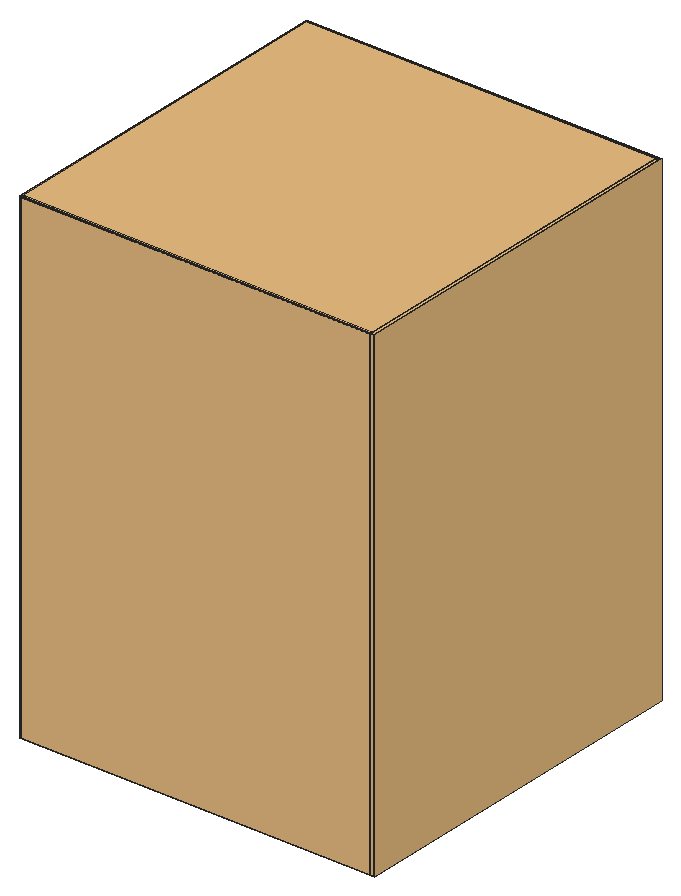
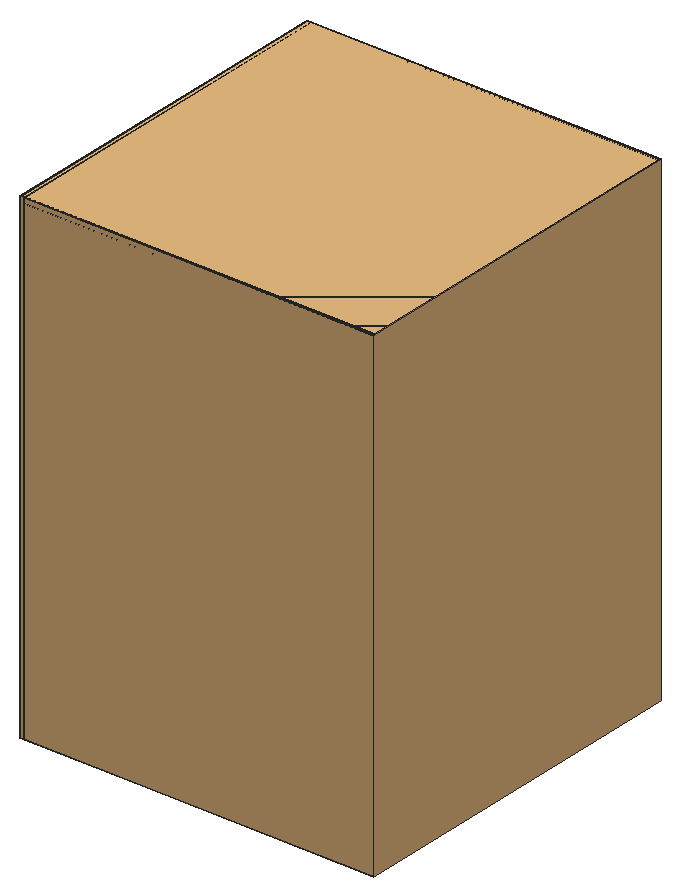
# SketchUp Ruby script. Lengths in inches.
U = 1.inch
M = Sketchup.active_model
def pt(a) = Geom::Point3d.new(a.map { |v| v * U })
def face(e, loops, mat)
  f = e.add_face(loops[0].map { |a| pt(a) })
  loops[1..].each { |l| e.add_face(l.map { |a| pt(a) }).erase! }
  f.material = f.back_material = mat if mat
  f
end
# faces: each face lists its corners as indices into pts; further lists are holes
def faces(e, pts, list, mat = nil) = list.each { |f| face(e, (f[0].is_a?(Array) ? f : [f]).map { |l| l.map { |i| pts[i] } }, mat) }
# xy, xz, yz: faces in a plane at the given z, y or x. An outline is a flat list of corners, or four numbers for a rectangle; further outlines are holes
def ring(l) = l.size == 4 ? [[l[0], l[1]], [l[2], l[1]], [l[2], l[3]], [l[0], l[3]]] : l.each_slice(2).to_a
def flat(e, list, mat, &to3) = list.each { |f| face(e, (f[0].is_a?(Array) ? f : [f]).map { |l| ring(l).map { |u, v| to3.(u, v) } }, mat) }
def xy(e, z, list, mat = nil) = flat(e, list, mat) { |x, y| [x, y, z] }
def xz(e, y, list, mat = nil) = flat(e, list, mat) { |x, z| [x, y, z] }
def yz(e, x, list, mat = nil) = flat(e, list, mat) { |y, z| [x, y, z] }
def lines(e, pts, list) = list.each { |a, b| e.add_line(pt(pts[a]), pt(pts[b])) }
# prism: a flat outline (further loops are holes) pulled along v
def prism(e, loops, v, mat = nil)
  f = face(e, loops, mat); d = Geom::Vector3d.new(v.map { |x| x * U })
  f.pushpull(f.normal.samedirection?(d) ? d.length : -d.length)
end
def box(e, o, s, mat = nil) = prism(e, [[o, [o[0] + s[0], o[1], o[2]], [o[0] + s[0], o[1] + s[1], o[2]], [o[0], o[1] + s[1], o[2]]]], [0, 0, s[2]], mat)
def at(x, y, z, deg = 0) = Geom::Transformation.translation(pt([x, y, z])) * Geom::Transformation.rotation(ORIGIN, Z_AXIS, deg.degrees)
def axes(o, x, y, z) = Geom::Transformation.new([*x, 0, *y, 0, *z, 0, *pt(o).to_a, 1])
def part(name) = M.definitions.add(name)
# library, detail: a bought-in or finely detailed component or shape, given as its bounding box
def library(name, o, s) = part(name).tap { |d| box(d.entities, o, s) }
def detail(e, o, s) = box(e.add_group.entities, o, s)
def put(e, d, t, mat = nil) = e.add_instance(d, t).tap { |i| i.material = mat if mat }
def group(e, t, mat = nil) = e.add_group.tap { |g| g.transformation = t; g.material = mat if mat }.entities
root = M.entities
M.materials.add("green").color = [174, 139, 102]
M.materials.add("vio").color = [206, 114, 100]
c1 = library("3DGeom~69_Defintion",[-21.55,-528.54,-60.47],[37.16,1000,121.53])
c2 = library("3DGeom~72_Defintion",[-21.55,-528.54,-60.94],[37.16,1000,122])
c3 = part("3DGeom~65_Defintion")
p = [[7.52,100.36,-59.99],[8.92,100.38,-59.73],[8.93,76.8125,-54.81],[7.56,76.76,-55.0625],[3.04,143.42,-39.85],[7.31,123.06,-53.64],
  [5.89,123.05,-53.91],[4.49,143.43,-39.59],[14.26,515.51,-51.87],[10.45,459.87,-31.05],[8.63,459.92,-31.36],[16.125,515.46,-51.55],
  [6.62,54.24,-42.53],[6.5,32.65,-26.04],[5.18,32.59,-26.27],[7.96,54.3,-42.28],[9.77,-132.64,-34.95],[8.22,-159.71,-27.66],
  [7.13,-159.66,-27.85],[10.89,-132.67,-34.76],[9.125,-89.93,-24.57],[11.4,-109.33,-33.07],[10.25,-109.31,-33.26],[10.29,-89.9375,-24.36],
  [-3.2,185.09,-5.2],[1.25,163.47,-22.06],[-0.23,163.47,-22.32],[-1.7,185.08,-4.93],[3.93,408.18,-14.71],[1.85,360.26,-1.6],
  [0.14,360.3,-1.9],[5.6875,408.13,-14.4],[2.8125,-189.42,-14.64],[-1.36,-221.25,2.05],[-2.375,-221.2,1.87],[3.87,-189.48,-14.46],
  [4.88,-58.05,-0.94],[8.29,-73.3125,-12.4],[7.1,-73.3125,-12.62],[6.08,-58.04,-0.72],[3.69,11.76,-9.89],[3.86,-8.04,3.3],
  [2.59,-8.09,3.07],[4.99,11.82,-9.66],[-2.72,316.3,7.07],[-3.06,276.15,12.48],[-4.67,276.18,12.21],[-1.0625,316.27,7.35],
  [2.27,-26.52,9.24],[4.32,-42.88,7.46],[3.09,-42.9,7.22],[3.52,-26.49,9.47],[-5.7,239.97,13.5],[-3.7,209.94,8.14],
  [-5.24,209.96,7.88],[-4.13,239.94,13.77],[-7.64,-254.13,18.93],[-11.22,-287.3125,33.93],[-12.17,-287.28,33.77],[-6.65,-254.18,19.09],
  [-15.18,-319.65,43.67],[-15.95,-351.88,49.35],[-16.84,-351.87,49.21],[-14.26,-319.67,43.82],[-17.57,-450.77,52.97],[-15.66,-484.48,50.06],
  [-16.4,-484.49,49.94],[-16.79,-450.76,53.09],[-17.79,-384.46,52.6],[-17.22,-417.43,53.99],[-18.03,-417.43,53.86],[-16.94,-384.47,52.74]]
faces(c3.entities,p,[[0,1,2],[0,2,3],[4,5,6],[4,7,5],[8,9,10],[8,11,9],[12,13,14],[12,15,13],
  [16,17,18],[16,19,17],[20,21,22],[20,23,21],[24,25,26],[24,27,25],[28,29,30],[28,31,29],
  [32,33,34],[32,35,33],[36,37,38],[36,39,37],[40,41,42],[40,43,41],[44,45,46],[44,47,45],
  [48,49,50],[48,51,49],[52,53,54],[52,55,53],[56,57,58],[56,59,57],[60,61,62],[60,63,61],
  [64,65,66],[64,67,65],[68,69,70],[68,71,69]],"green")
c4 = part("3DGeom~68_Defintion")
p = [[6.16,100.31,-59.87],[7.52,100.34,-59.98],[7.56,76.74,-55.05],[6.21,76.79,-54.96],[8.91,100.36,-59.72],[10.17,76.95,-54.21],
  [8.92,76.8,-54.8],[10.1875,100.38,-59.09],[1.63,143.2,-39.79],[5.89,123.02,-53.9],[4.5,122.88,-53.81],[3.04,143.39,-39.84],
  [4.48,143.4,-39.58],[8.62,122.92,-53.03],[7.31,123.04,-53.63],[5.83,143.21,-39.01],[12.45,515.58,-51.71],[14.26,515.4,-51.86],
  [8.63,459.82,-31.36],[6.87,459.98,-31.21],[16.12,515.35,-51.54],[12.12,459.84,-30.29],[10.44,459.77,-31.05],[17.84,515.4375,-50.76],
  [5.3,54.32,-42.45],[6.61,54.23,-42.52],[5.18,32.58,-26.27],[3.89,32.68,-26.21],[7.96,54.29,-42.28],[7.71,32.88,-25.52],
  [6.5,32.65,-26.03],[9.1875,54.5,-41.73],[7.71,32.88,-25.52],[8.67,-132.56,-34.83],[9.76,-132.61,-34.94],[7.13,-159.63,-27.84],
  [10.89,-132.65,-34.76],[9.23,-159.65,-27.2],[8.22,-159.68,-27.66],[6.07,-159.51,-27.75],[11.93,-132.65,-34.28],[7.99,-90.02,-24.49],
  [9.125,-89.91,-24.56],[10.25,-109.28,-33.26],[9.13,-109.32,-33.15],[10.29,-89.92,-24.36],[12.45,-109.39,-32.58],[11.4,-109.31,-33.07],
  [11.37,-90.05,-23.89],[-4.67,184.89,-5.11],[-0.23,163.4375,-22.32],[-1.66,163.24,-22.26],[-3.2,185.05,-5.19],[-1.7,185.04,-4.93],
  [2.62,163.24,-21.49],[1.25,163.44,-22.05],[-0.3,184.86,-4.34],[2.62,163.24,-21.49],[2.21,408.23,-14.55],[3.93,408.09,-14.7],
  [0.14,360.23,-1.9],[1.79,-189.24,-14.5625],[-2.375,-221.15,1.87],[-3.36,-221.01,1.9375],[2.8125,-189.38,-14.64],[-1.53,360.34,-1.74],
  [3.87,-189.4375,-14.46],[-0.41,-221.16,2.46],[-1.36,-221.21,2.05],[4.84,-189.4,-14.02],[5.6875,408.05,-14.4],[3.43,360.23,-0.88],
  [1.85,360.1875,-1.6],[7.3125,408.11,-13.66],[3.71,-58.1875,-0.89],[7.1,-73.3,-12.61],[5.95,-73.45,-12.5625],[4.88,-58.04,-0.94],
  [6.08,-58.03,-0.72],[9.39,-73.45,-11.9375],[8.29,-73.3,-12.4],[7.2,-58.16,-0.23],[9.39,-73.45,-11.9375],[2.43,11.85,-9.83],
  [3.69,11.75,-9.89],[2.59,-8.09,3.07],[1.34,-8.02,3.15],[4.99,11.82,-9.66],[5.02,-7.87,3.83],[3.86,-8.04,3.3],
  [6.17,12.03,-9.14],[5.02,-7.87,3.83],[-4.34,316.32,7.22],[-2.72,316.23,7.07],[-4.67,276.12,12.2],[1.05,-26.51,9.34],
  [3.09,-42.89,7.22],[1.89,-42.99,7.31],[2.27,-26.51,9.24],[-6.24,276.17,12.36],[-1.0625,316.2,7.35],[-1.57,276.09,13.17],
  [-3.06,276.09,12.48],[0.47,316.22,8.0625],[3.52,-26.49,9.47],[5.44,-42.94,7.99],[4.32,-42.875,7.45],[-7.22,239.93,13.65],
  [-5.23,209.91,7.88],[-6.73,209.82,8.01],[-5.69,239.92,13.5],[4.65,-26.43,10.03],[-4.13,239.89,13.76],[-2.29,209.78,8.79],
  [-3.7,209.9,8.14],[-2.7,239.86,14.43],[-8.59,-253.95,18.99],[-7.64,-254.08,18.92],[-12.17,-287.22,33.76],[-13.09,-287.11,33.84],
  [-6.65,-254.125,19.09],[-10.33,-287.22,34.3125],[-11.21,-287.25,33.92],[-5.74,-254.08,19.49],[-16.07,-319.53,43.75],[-15.17,-319.59,43.66],
  [-16.83,-351.79,49.2],[-17.69,-351.76,49.29],[-14.26,-319.61,43.81],[-15.14,-351.79,49.71],[-15.95,-351.81,49.34],[-13.41,-319.59,44.19],
  [-18.32,-450.69,53.04],[-17.57,-450.68,52.96],[-16.4,-484.39,49.93],[-17.12,-484.42,50.01],[-16.79,-450.67,53.08],[-14.97,-484.38,50.36],
  [-15.66,-484.375,50.05],[-16.08,-450.67,53.41],[-18.61,-384.37,52.68],[-17.78,-384.38,52.59],[-18.03,-417.34,53.85],[-18.82,-417.34,53.93],
  [-16.9375,-384.39,52.73],[-16.47,-417.34,54.32],[-17.22,-417.34,53.98],[-16.16,-384.38,53.08]]
faces(c4.entities,p,[[0,1,2],[0,2,3],[4,5,6],[4,7,5],[8,9,10],[8,11,9],[12,13,14],[12,15,13],
  [16,17,18],[16,18,19],[20,21,22],[20,23,21],[24,25,26],[24,26,27],[28,29,30],[28,31,32],
  [33,34,35],[36,37,38],[33,35,39],[36,40,37],[41,42,43],[41,43,44],[45,46,47],[45,48,46],
  [49,50,51],[49,52,50],[53,54,55],[53,56,57],[58,59,60],[61,62,63],[61,64,62],[58,60,65],
  [66,67,68],[66,69,67],[70,71,72],[70,73,71],[74,75,76],[74,77,75],[78,79,80],[78,81,82],
  [83,84,85],[83,85,86],[87,88,89],[87,90,91],[92,93,94],[95,96,97],[95,98,96],[92,94,99],
  [100,101,102],[100,103,101],[104,105,106],[107,108,109],[107,110,108],[104,111,105],[112,113,114],[112,115,113],
  [116,117,118],[116,118,119],[120,121,122],[120,123,121],[124,125,126],[124,126,127],[128,129,130],[128,131,129],
  [132,133,134],[132,134,135],[136,137,138],[136,139,137],[140,141,142],[140,142,143],[144,145,146],[144,147,145]],"green")
c5 = library("3DGeom~67_Defintion",[-21.08,-482.92,-59.16],[42.16,1000,118.9])
c6 = library("3DGeom~71_Defintion",[-21.08,-482.92,-59.62],[42.16,1000,119.36])
c7 = part("3DGeom~73_Defintion")
p = [[11.99,496.51,-49.8],[15.53,496.29,-49.63],[13.73,496.34,-49.94],[11.99,496.51,-49.8],[19.55,496.875,-46.43],[15.53,496.29,-49.63],
  [8.98,497.16,-48.31],[19.55,496.875,-46.43],[11.99,496.51,-49.8],[8.98,497.16,-48.31],[11.99,496.51,-49.8],[10.38,496.79,-49.24],
  [15.53,496.29,-49.63],[19.55,496.875,-46.43],[18.54,496.57,-47.79],[15.53,496.29,-49.63],[18.54,496.57,-47.79],[17.18,496.37,-48.89],
  [7.13,498.09,-45.48],[19.55,496.875,-46.43],[8.98,497.16,-48.31],[7.13,498.09,-45.48],[8.98,497.16,-48.31],[7.87,497.6,-47.04],
  [7.06,499.03,-42.12],[19.55,496.875,-46.43],[7.13,498.09,-45.48],[8.7,499.72,-39.2],[19.55,496.875,-46.43],[7.06,499.03,-42.12],
  [11.72,500,-37.36],[19.55,496.875,-46.43],[8.7,499.72,-39.2],[15.25,499.78,-37.19],[19.55,496.875,-46.43],[11.72,500,-37.36],
  [20.18,497.26,-44.875],[19.55,496.875,-46.43],[15.25,499.78,-37.19],[7.06,499.03,-42.12],[7.13,498.09,-45.48],[6.86,498.58,-43.78],
  [20.18,497.26,-44.875],[15.25,499.78,-37.19],[16.86,499.5,-37.75],[19.37,498.7,-39.95],[20.18,497.26,-44.875],[16.86,499.5,-37.75],
  [20.11,498.2,-41.51],[20.18,497.26,-44.875],[19.37,498.7,-39.95],[20.11,498.2,-41.51],[20.38,497.71,-43.21],[20.18,497.26,-44.875],
  [8.7,499.72,-39.2],[7.06,499.03,-42.12],[7.6875,499.41,-40.5625],[19.37,498.7,-39.95],[16.86,499.5,-37.75],[18.26,499.13,-38.68],
  [11.72,500,-37.36],[8.7,499.72,-39.2],[10.0625,499.92,-38.11],[15.25,499.78,-37.19],[11.72,500,-37.36],[13.51,499.95,-37.05],
  [-14.64,-499.34,43.17],[-13.98,-499.3,43.1],[-13.3,-499.28,43.21],[-15.79,-499.47,43.77],[-15.26,-499.4,43.4],[-14.64,-499.34,43.17],
  [-15.79,-499.47,43.77],[-14.64,-499.34,43.17],[-11.78,-499.375,44.44],[-14.64,-499.34,43.17],[-13.3,-499.28,43.21],[-11.78,-499.375,44.44],
  [-13.3,-499.28,43.21],[-12.16,-499.32,43.91],[-11.78,-499.375,44.44],[-13.3,-499.28,43.21],[-12.68,-499.29,43.49],[-12.16,-499.32,43.91],
  [-16.49,-499.66,44.89],[-16.21,-499.56,44.28],[-15.79,-499.47,43.77],[-16.49,-499.66,44.89],[-15.79,-499.47,43.77],[-11.78,-499.375,44.44],
  [-15.9,-499.96,47.36],[-16.52,-499.84,46.22],[-11.78,-499.375,44.44],[-14.76,-500,48.06],[-15.9,-499.96,47.36],[-11.78,-499.375,44.44],
  [-13.42,-499.94,48.1],[-14.76,-500,48.06],[-11.78,-499.375,44.44],[-11.54,-499.44,45.05],[-13.42,-499.94,48.1],[-11.78,-499.375,44.44],
  [-16.52,-499.84,46.22],[-16.49,-499.66,44.89],[-11.78,-499.375,44.44],[-16.52,-499.84,46.22],[-16.6,-499.75,45.57],[-16.49,-499.66,44.89],
  [-11.54,-499.44,45.05],[-12.81,-499.88,47.87],[-13.42,-499.94,48.1],[-11.85,-499.72,46.99],[-12.81,-499.88,47.87],[-11.54,-499.44,45.05],
  [-11.54,-499.44,45.05],[-11.57,-499.625,46.375],[-11.85,-499.72,46.99],[-11.54,-499.44,45.05],[-11.47,-499.53,45.7],[-11.57,-499.625,46.375],
  [-15.9,-499.96,47.36],[-16.28,-499.91,46.83],[-16.52,-499.84,46.22],[-11.85,-499.72,46.99],[-12.28,-499.81,47.5],[-12.81,-499.88,47.87],
  [-14.76,-500,48.06],[-15.39,-499.99,47.78],[-15.9,-499.96,47.36],[-13.42,-499.94,48.1],[-14.08,-499.98,48.17],[-14.76,-500,48.06]]
faces(c7.entities,p,[[0,1,2],[3,4,5],[6,7,8],[9,10,11],[12,13,14],[15,16,17],[18,19,20],[21,22,23],
  [24,25,26],[27,28,29],[30,31,32],[33,34,35],[36,37,38],[39,40,41],[42,43,44],[45,46,47],
  [48,49,50],[51,52,53],[54,55,56],[57,58,59],[60,61,62],[63,64,65],[66,67,68],[69,70,71],
  [72,73,74],[75,76,77],[78,79,80],[81,82,83],[84,85,86],[87,88,89],[90,91,92],[93,94,95],
  [96,97,98],[99,100,101],[102,103,104],[105,106,107],[108,109,110],[111,112,113],[114,115,116],[117,118,119],
  [120,121,122],[123,124,125],[126,127,128],[129,130,131]],"green")
c8 = library("3DGeom~1_Defintion",[-369.63,-500,-363.56],[735.81,1000,728.59])
c9 = library("3DGeom~2_Defintion",[-372.64,-496.69,-369.59],[746.89,1000,738.52])
c10 = library("3DGeom~3_Defintion",[-370.01,-499.5,-356.78],[740.02,1000,722.18])
c11 = library("3DGeom~4_Defintion",[-369.63,-500,-365.03],[739.26,1000,729.3])
c12 = library("3DGeom~5_Defintion",[-370.16,-506.05,-369.45],[742.08,1000,738.24])
c13 = library("3DGeom~6_Defintion",[-367.72,-498.8,-365.91],[735.57,1000,731.94])
c14 = part("3DGeom~242_Defintion")
p = [[-230.85,-87.93,-431.85],[22.11,-101.53,-485.51],[16.43,-294.21,-360.73],[264.23,-254.8,-301.01],[16.43,-294.21,-360.73],[269.15,-87.93,-409.08],
  [264.23,-254.8,-301.01],[-231.0625,102.5,-427.26],[21.87,118.36,-480.21],[-230.85,-87.93,-431.85],[268.9375,102.5,-404.49],[-236.35,265.46,-311.23],
  [15.77,306.53,-346.23],[-236.35,265.46,-311.23],[-230.85,-87.93,-431.85],[16.43,-294.21,-360.73],[-235.78,-254.8,-323.78],[-421.96,-50.77,-262.47],
  [-230.85,-87.93,-431.85],[-235.78,-254.8,-323.78],[-422.08,59.18,-259.82],[-230.85,-87.93,-431.85],[-422.08,59.18,-259.82],[-230.85,-87.93,-431.85],
  [-421.96,-50.77,-262.47],[-425.13,153.27,-192.83],[-231.0625,102.5,-427.26],[-422.08,59.18,-259.82],[-236.35,265.46,-311.23],[-231.0625,102.5,-427.26],
  [269.15,-87.93,-409.08],[441.23,-147.11,-160.65],[264.23,-254.8,-301.01],[269.15,-87.93,-409.08],[444.07,-50.76,-223.04],[268.9375,102.5,-404.49],
  [269.15,-87.93,-409.08],[268.9375,102.5,-404.49],[443.95,59.18,-220.39],[263.65,265.47,-288.46],[268.9375,102.5,-404.49],[263.65,265.47,-288.46],
  [-235.78,-254.8,-323.78],[16.43,-294.21,-360.73],[6.34,-408.0625,-139.28],[255.49,-353.39,-109.24],[264.23,-254.8,-301.01],[-245.29,357.3,-114.86],
  [15.77,306.53,-346.23],[-236.35,265.46,-311.23],[5.44,412.57,-119.48],[263.65,265.47,-288.46],[15.77,306.53,-346.23],[-245.29,357.3,-114.86],
  [15.77,306.53,-346.23],[-235.78,-254.8,-323.78],[-244.51,-353.39,-132.01],[-424.8,-147.11,-200.08],[-244.51,-353.39,-132.01],[-430.29,206.29,-79.46],
  [-245.29,357.3,-114.86],[264.23,-254.8,-301.01],[436.18,-204.03,-49.92],[255.49,-353.39,-109.24],[264.23,-254.8,-301.01],[263.65,265.47,-288.46],
  [440.9,153.27,-153.4],[254.71,357.3,-92.09],[263.65,265.47,-288.46],[254.71,357.3,-92.09],[263.65,265.47,-288.46],[-500,0,-22.77],
  [500,0,22.77],[-429.84,-204.03,-89.36],[435.73,206.29,-40.02],[254.71,357.3,-92.09],[-244.51,-353.39,-132.01],[-5.44,-412.57,119.48],
  [245.29,-357.3,114.86],[-244.51,-353.39,-132.01],[-254.71,-357.3,92.09],[-254.71,-357.3,92.09],[-255.49,353.39,109.24],[-6.34,408.0625,139.28],
  [-255.49,353.39,109.24],[-245.29,357.3,-114.86],[-436.18,204.03,49.92],[-255.49,353.39,109.24],[255.49,-353.39,-109.24],[430.29,-206.29,79.46],
  [245.29,-357.3,114.86],[255.49,-353.39,-109.24],[244.51,353.39,132.01],[254.71,357.3,-92.09],[244.51,353.39,132.01],[-435.73,-206.29,40.02],
  [429.84,204.03,89.36],[244.51,353.39,132.01],[-440.9,-153.27,153.4],[-443.95,-59.18,220.39],[-444.07,50.77,223.04],[-441.23,147.11,160.65],
  [425.13,-153.27,192.83],[422.08,-59.18,259.82],[421.96,50.77,262.47],[424.8,147.11,200.08],[-263.65,-265.47,288.46],[245.29,-357.3,114.86],
  [235.78,254.8,323.78],[235.78,254.8,323.78],[244.51,353.39,132.01],[-254.71,-357.3,92.09],[-15.77,-306.53,346.23],[-254.71,-357.3,92.09],
  [-15.77,-306.53,346.23],[-263.65,-265.47,288.46],[-264.22,254.8,301.01],[-264.22,254.8,301.01],[-255.49,353.39,109.24],[236.35,-265.47,311.23],
  [245.29,-357.3,114.86],[236.35,-265.47,311.23],[236.35,-265.47,311.23],[-15.77,-306.53,346.23],[-16.43,294.21,360.73],[235.78,254.8,323.78],
  [-264.22,254.8,301.01],[-268.9375,-102.5,404.49],[236.35,-265.47,311.23],[230.85,87.93,431.85],[230.85,87.93,431.85],[235.78,254.8,323.78],
  [-269.15,87.93,409.08],[236.35,-265.47,311.23],[231.0625,-102.5,427.26],[231.0625,-102.5,427.26],[422.08,-59.18,259.82],[421.96,50.77,262.47],
  [421.96,50.77,262.47],[230.85,87.93,431.85],[-263.65,-265.47,288.46],[-15.77,-306.53,346.23],[-21.87,-118.36,480.21],[-263.65,-265.47,288.46],
  [-268.9375,-102.5,404.49],[-269.15,87.93,409.08],[-16.43,294.21,360.73],[-264.22,254.8,301.01],[236.35,-265.47,311.23],[-22.11,101.53,485.51],
  [235.78,254.8,323.78],[235.78,254.8,323.78],[-16.43,294.21,360.73],[-269.15,87.93,409.08],[-16.43,294.21,360.73],[-268.9375,-102.5,404.49],
  [-268.9375,-102.5,404.49],[-269.15,87.93,409.08]]
faces(c14.entities,p,[[0,1,2],[1,3,4],[1,5,6],[7,8,1],[7,1,9],[8,5,1],[8,10,5],[11,8,7],
  [12,10,8],[13,12,8],[14,15,16],[17,18,19],[20,7,21],[22,23,24],[25,26,27],[25,28,29],
  [30,31,32],[33,34,31],[35,34,36],[37,38,34],[39,38,40],[12,41,10],[42,43,44],[43,45,44],
  [43,46,45],[47,48,49],[50,51,52],[53,50,54],[55,44,56],[57,19,58],[17,19,57],[59,28,25],
  [59,60,28],[61,62,63],[64,31,62],[65,66,38],[67,66,68],[50,69,70],[17,57,71],[27,17,71],
  [25,27,71],[31,34,72],[34,38,72],[38,66,72],[57,58,73],[57,73,71],[59,25,71],[62,31,72],
  [66,74,72],[75,74,66],[76,44,77],[44,78,77],[44,45,78],[79,77,80],[73,58,81],[82,83,50],
  [84,50,85],[83,69,50],[86,87,60],[86,60,59],[88,89,90],[91,62,89],[92,74,93],[83,94,69],
  [73,81,95],[73,95,71],[86,59,71],[89,62,72],[74,96,72],[97,96,74],[95,98,71],[98,99,71],
  [99,100,71],[101,86,71],[100,101,71],[102,89,72],[103,102,72],[104,103,72],[105,104,72],[96,105,72],
  [95,81,106],[95,106,98],[101,87,86],[107,89,102],[108,105,96],[109,96,110],[111,77,112],[113,114,115],
  [101,116,87],[117,83,118],[77,78,119],[120,102,121],[77,122,123],[124,125,94],[124,94,83],[126,124,83],
  [98,106,127],[98,127,99],[100,116,101],[128,102,103],[129,104,105],[130,105,131],[99,127,132],[99,132,100],
  [100,132,116],[133,103,134],[135,136,137],[135,138,139],[140,141,142],[143,142,144],[145,146,147],[141,148,135],
  [149,139,150],[149,151,152],[141,135,142],[153,149,154],[155,142,149],[156,149,157],[142,135,139],[142,139,149]],"vio")
c15 = part("3DGeom~216_Defintion")
p = [[-234.26,0,-442.1],[18.17,0,-500],[15.74,-212.36,-433.01],[263.63,-183.91,-365.91],[265.74,0,-423.93],[-236.37,183.91,-384.09],
  [15.74,212.36,-433.01],[-236.37,-183.91,-384.09],[-423.93,0,-265.74],[-236.37,-183.91,-384.09],[-425.14,106.18,-232.25],[-425.14,106.18,-232.25],
  [-423.93,0,-265.74],[-236.37,-183.91,-384.09],[9.09,-367.82,-250],[257.87,-318.54,-207.42],[9.09,-367.82,-250],[257.87,-318.54,-207.42],
  [263.63,183.91,-365.91],[-242.13,318.54,-225.59],[9.09,367.82,-250],[-242.13,318.54,-225.59],[265.74,0,-423.93],[440.88,-106.18,-200.77],
  [263.63,-183.91,-365.91],[265.74,0,-423.93],[442.1,0,-234.26],[263.63,183.91,-365.91],[265.74,0,-423.93],[-236.37,-183.91,-384.09],
  [9.09,-367.82,-250],[-242.13,-318.54,-225.59],[-425.14,-106.18,-232.25],[-236.37,-183.91,-384.09],[-242.13,-318.54,-225.59],[-423.93,0,-265.74],
  [-236.37,-183.91,-384.09],[-425.14,-106.18,-232.25],[-428.47,183.91,-140.74],[-236.37,183.91,-384.09],[-425.14,106.18,-232.25],[-242.13,318.54,-225.59],
  [-236.37,183.91,-384.09],[263.63,-183.91,-365.91],[437.56,-183.91,-109.26],[257.87,-318.54,-207.42],[263.63,-183.91,-365.91],[263.63,183.91,-365.91],
  [440.88,106.18,-200.77],[257.87,318.54,-207.42],[263.63,183.91,-365.91],[257.87,318.54,-207.42],[-423.93,0,-265.74],[-500,0,-18.17],
  [-242.13,-318.54,-225.59],[9.09,-367.82,-250],[0,-424.72,0],[250,-367.82,9.09],[257.87,-318.54,-207.42],[-250,367.82,-9.09],
  [9.09,367.82,-250],[-242.13,318.54,-225.59],[0,424.72,0],[257.87,318.54,-207.42],[9.09,367.82,-250],[-250,367.82,-9.09],
  [9.09,367.82,-250],[500,0,18.17],[-428.47,-183.91,-140.74],[-242.13,-318.54,-225.59],[-250,-367.82,-9.09],[-250,-367.82,-9.09],
  [-433.01,212.36,-15.74],[-250,367.82,-9.09],[257.87,-318.54,-207.42],[433.01,-212.36,15.74],[250,-367.82,9.09],[257.87,-318.54,-207.42],
  [257.87,318.54,-207.42],[437.56,183.91,-109.26],[250,367.82,9.09],[257.87,318.54,-207.42],[250,367.82,9.09],[257.87,318.54,-207.42],
  [-433.01,-212.36,-15.74],[433.01,212.36,15.74],[250,367.82,9.09],[-437.56,-183.91,109.26],[-440.88,-106.18,200.77],[-442.1,0,234.26],
  [-437.56,183.91,109.26],[-440.88,106.18,200.77],[-257.87,-318.54,207.42],[-250,-367.82,-9.09],[-9.09,-367.82,250],[-250,-367.82,-9.09],
  [-9.09,-367.82,250],[-257.87,-318.54,207.42],[-257.87,318.54,207.42],[-257.87,318.54,207.42],[-250,367.82,-9.09],[242.13,-318.54,225.59],
  [-9.09,-367.82,250],[242.13,-318.54,225.59],[-257.87,318.54,207.42],[-9.09,367.82,250],[250,-367.82,9.09],[428.47,-183.91,140.74],
  [242.13,-318.54,225.59],[250,-367.82,9.09],[242.13,318.54,225.59],[250,367.82,9.09],[242.13,318.54,225.59],[428.47,183.91,140.74],
  [242.13,318.54,225.59],[425.14,-106.18,232.25],[423.93,0,265.74],[425.14,-106.18,232.25],[425.14,106.18,232.25],[423.93,0,265.74],
  [-263.63,-183.91,365.91],[242.13,-318.54,225.59],[425.14,-106.18,232.25],[236.37,183.91,384.09],[236.37,183.91,384.09],[242.13,318.54,225.59],
  [-265.74,0,423.93],[-263.63,183.91,365.91],[-257.87,-318.54,207.42],[-9.09,-367.82,250],[-15.74,-212.36,433.01],[-257.87,-318.54,207.42],
  [-263.63,-183.91,365.91],[-263.63,183.91,365.91],[-9.09,367.82,250],[-257.87,318.54,207.42],[242.13,-318.54,225.59],[236.37,-183.91,384.09],
  [242.13,-318.54,225.59],[425.14,-106.18,232.25],[236.37,-183.91,384.09],[-15.74,212.36,433.01],[236.37,183.91,384.09],[242.13,318.54,225.59],
  [-9.09,367.82,250],[425.14,-106.18,232.25],[423.93,0,265.74],[234.26,0,442.1],[425.14,106.18,232.25],[425.14,106.18,232.25],
  [-263.63,183.91,365.91],[-9.09,367.82,250],[-263.63,-183.91,365.91],[-18.17,0,500],[-263.63,-183.91,365.91],[-265.74,0,423.93],
  [-265.74,0,423.93],[-263.63,183.91,365.91],[-265.74,0,423.93]]
faces(c15.entities,p,[[0,1,2],[1,3,2],[1,4,3],[5,6,1],[5,1,0],[6,4,1],[0,2,7],[8,0,9],
  [10,5,0],[11,0,12],[13,2,14],[2,15,16],[2,3,17],[6,18,4],[19,6,5],[20,18,6],
  [21,20,6],[22,23,24],[25,26,23],[27,26,28],[29,30,31],[32,33,34],[35,36,37],[38,39,40],
  [38,41,42],[43,44,45],[46,23,44],[47,48,26],[49,48,50],[20,51,18],[52,32,53],[40,52,53],
  [54,55,56],[55,57,56],[55,58,57],[59,60,61],[62,63,64],[65,62,66],[23,26,67],[26,48,67],
  [32,34,68],[32,68,53],[38,40,53],[69,56,70],[68,34,71],[72,41,38],[72,73,41],[74,75,76],
  [77,44,75],[78,79,48],[80,79,81],[62,82,83],[44,23,67],[48,79,67],[68,71,84],[68,84,53],
  [72,38,53],[75,44,67],[79,85,67],[86,85,79],[84,87,53],[87,88,53],[88,89,53],[90,72,53],
  [91,90,53],[89,91,53],[84,71,92],[84,92,87],[90,73,72],[93,56,94],[95,96,97],[90,98,73],
  [99,62,100],[56,101,102],[56,57,103],[104,105,62],[105,82,62],[106,107,108],[109,75,107],[110,85,111],
  [105,112,82],[107,75,67],[85,113,67],[114,113,85],[115,107,67],[116,117,67],[118,119,67],[113,118,67],
  [87,92,120],[87,120,88],[91,98,90],[121,107,122],[123,118,113],[124,113,125],[88,120,126],[88,126,89],
  [89,127,91],[91,127,98],[128,129,130],[131,130,132],[133,134,135],[129,136,137],[138,139,140],[141,142,143],
  [141,143,144],[137,145,146],[147,146,148],[147,149,142],[89,126,127],[129,137,130],[150,141,151],[137,146,147],
  [152,130,153],[154,153,155],[156,141,157],[130,137,147],[153,147,142],[153,142,141],[158,153,141],[130,147,153]],"vio")
c16 = library("3DGeom~90_Defintion",[-21.63,-500,-162.35],[43.26,1000,324.7])
c17 = part("3DGeom~91_Defintion")
p = [[4.77,500,-131.64],[5.88,490.68,-162.35],[-2.34,491.3,-160.59],[4.77,500,-131.64],[13.96,491.3,-160],[5.88,490.68,-162.35],
  [4.77,500,-131.64],[-2.34,491.3,-160.59],[-8.52,493.01,-155.1875],[4.77,500,-131.64],[19.73,493.01,-154.16],[13.96,491.3,-160],
  [4.77,500,-131.64],[-8.52,493.01,-155.1875],[-10.98,495.34,-147.59],[4.77,500,-131.64],[21.63,495.34,-146.41],[19.73,493.01,-154.16],
  [4.77,500,-131.64],[-10.98,495.34,-147.59],[-9.08,497.67,-139.83],[4.77,500,-131.64],[19.17,497.67,-138.81],[21.63,495.34,-146.41],
  [4.77,500,-131.64],[-9.08,497.67,-139.83],[-3.3125,499.375,-134],[4.77,500,-131.64],[13,499.375,-133.4],[19.17,497.67,-138.81],
  [-4.37,-494.09,119.72],[-5.53,-500,151.58],[-18.78,-495.57,127.17],[9.46,-495.57,128.2],[-5.53,-500,151.58],[-4.37,-494.09,119.72],
  [-4.37,-494.09,119.72],[-18.78,-495.57,127.17],[-12.6,-494.49,121.56],[9.46,-495.57,128.2],[-4.37,-494.09,119.72],[3.71,-494.49,122.15],
  [-18.78,-495.57,127.17],[-5.53,-500,151.58],[-19.36,-498.52,143.1],[-18.78,-495.57,127.17],[-19.36,-498.52,143.1],[-21.25,-497.04,135.06],
  [8.89,-498.52,144.13],[-5.53,-500,151.58],[9.46,-495.57,128.2],[8.89,-498.52,144.13],[9.46,-495.57,128.2],[11.36,-497.04,136.24],
  [-5.53,-500,151.58],[-13.6,-499.6,149.15],[-19.36,-498.52,143.1],[-5.53,-500,151.58],[8.89,-498.52,144.13],[2.7,-499.6,149.74]]
faces(c17.entities,p,[[0,1,2],[3,4,5],[6,7,8],[9,10,11],[12,13,14],[15,16,17],[18,19,20],[21,22,23],
  [24,25,26],[27,28,29],[30,31,32],[33,34,35],[36,37,38],[39,40,41],[42,43,44],[45,46,47],
  [48,49,50],[51,52,53],[54,55,56],[57,58,59]],"green")
put(root,c1,axes([14.0625,134.46,36.46],[0,0.01017,0],[0,0,-0.01017],[-0.01017,0,0]),"green")
put(root,c2,axes([14.0625,134.46,36.46],[0,0.01017,0],[0,0,-0.01017],[-0.01017,0,0]),"green")
put(root,c3,axes([14.0625,134.46,36.46],[0,0.01036,0],[0,0,-0.01036],[-0.01036,0,0]),"green")
put(root,c4,axes([14.0625,134.46,36.46],[0,0.01036,0],[0,0,-0.01036],[-0.01036,0,0]),"green")
put(root,c5,axes([14.0625,134.46,36.46],[0,0.0104,0],[0,0,-0.0104],[-0.0104,0,0]),"green")
put(root,c6,axes([14.0625,134.46,36.46],[0,0.0104,0],[0,0,-0.0104],[-0.0104,0,0]),"green")
put(root,c7,axes([14.0625,134.46,36.46],[0,0.01076,0],[0,0,-0.01076],[-0.01076,0,0]),"green")
g1 = group(root,at(15.3125,134.49,26.21))
put(g1,c8,axes([-1.67,0,10.71],[0,0.0107,0],[0,0,-0.0107],[-0.0107,0,0]),"green")
put(g1,c9,axes([-1.67,0,10.71],[0,0.01056,0],[0,0,-0.01056],[-0.01056,0,0]),"green")
put(g1,c10,axes([-1.67,0,10.71],[0,0.01069,0],[0,0,-0.01069],[-0.01069,0,0]),"green")
put(g1,c11,axes([-1.67,0,10.71],[0,0.0107,0],[0,0,-0.0107],[-0.0107,0,0]),"green")
put(g1,c12,axes([-1.67,0,10.71],[0,0.01057,0],[0,0,-0.01057],[-0.01057,0,0]),"green")
put(g1,c13,axes([-1.67,0,10.71],[0,0.01067,0],[0,0,-0.01067],[-0.01067,0,0]),"green")
g2 = group(root,at(15.3125,134.49,26.21))
put(g2,c14,axes([-1.86,0.02,7.01],[0,0.00039,0],[0,0,-0.00039],[-0.00039,0,0]),"vio")
g3 = group(root,at(15.3125,134.49,26.21))
put(g3,c15,axes([-1.32,0.04,6.71],[0,0.00039,0],[0,0,-0.00039],[-0.00039,0,0]),"vio")
g4 = group(root,at(15.3125,134.49,26.21))
put(g4,c16,axes([-1.19,0.04,6.22],[0,0.00091,0],[0,0,-0.00091],[-0.00091,0,0]),"green")
put(g4,c17,axes([-1.19,0.04,6.22],[0,0.00091,0],[0,0,-0.00091],[-0.00091,0,0]),"green")
